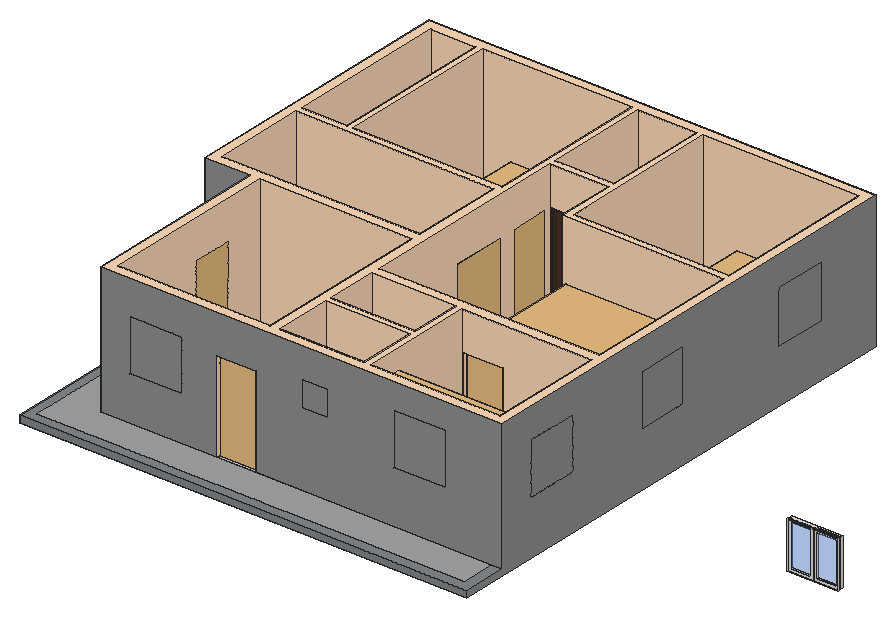
# SketchUp Ruby script. Lengths in inches.
U = 1.inch
M = Sketchup.active_model
def pt(a) = Geom::Point3d.new(a.map { |v| v * U })
def face(e, loops, mat)
  f = e.add_face(loops[0].map { |a| pt(a) })
  loops[1..].each { |l| e.add_face(l.map { |a| pt(a) }).erase! }
  f.material = f.back_material = mat if mat
  f
end
# faces: each face lists its corners as indices into pts; further lists are holes
def faces(e, pts, list, mat = nil) = list.each { |f| face(e, (f[0].is_a?(Array) ? f : [f]).map { |l| l.map { |i| pts[i] } }, mat) }
# xy, xz, yz: faces in a plane at the given z, y or x. An outline is a flat list of corners, or four numbers for a rectangle; further outlines are holes
def ring(l) = l.size == 4 ? [[l[0], l[1]], [l[2], l[1]], [l[2], l[3]], [l[0], l[3]]] : l.each_slice(2).to_a
def flat(e, list, mat, &to3) = list.each { |f| face(e, (f[0].is_a?(Array) ? f : [f]).map { |l| ring(l).map { |u, v| to3.(u, v) } }, mat) }
def xy(e, z, list, mat = nil) = flat(e, list, mat) { |x, y| [x, y, z] }
def xz(e, y, list, mat = nil) = flat(e, list, mat) { |x, z| [x, y, z] }
def yz(e, x, list, mat = nil) = flat(e, list, mat) { |y, z| [x, y, z] }
def lines(e, pts, list) = list.each { |a, b| e.add_line(pt(pts[a]), pt(pts[b])) }
# prism: a flat outline (further loops are holes) pulled along v
def prism(e, loops, v, mat = nil)
  f = face(e, loops, mat); d = Geom::Vector3d.new(v.map { |x| x * U })
  f.pushpull(f.normal.samedirection?(d) ? d.length : -d.length)
end
def box(e, o, s, mat = nil) = prism(e, [[o, [o[0] + s[0], o[1], o[2]], [o[0] + s[0], o[1] + s[1], o[2]], [o[0], o[1] + s[1], o[2]]]], [0, 0, s[2]], mat)
def at(x, y, z, deg = 0) = Geom::Transformation.translation(pt([x, y, z])) * Geom::Transformation.rotation(ORIGIN, Z_AXIS, deg.degrees)
def axes(o, x, y, z) = Geom::Transformation.new([*x, 0, *y, 0, *z, 0, *pt(o).to_a, 1])
def part(name) = M.definitions.add(name)
# library, detail: a bought-in or finely detailed component or shape, given as its bounding box
def library(name, o, s) = part(name).tap { |d| box(d.entities, o, s) }
def detail(e, o, s) = box(e.add_group.entities, o, s)
def put(e, d, t, mat = nil) = e.add_instance(d, t).tap { |i| i.material = mat if mat }
def group(e, t, mat = nil) = e.add_group.tap { |g| g.transformation = t; g.material = mat if mat }.entities
root = M.entities
M.materials.add("Polis06_194").color = [79, 50, 36]
M.materials.add("[0027_PeachPuff]").color = [255, 218, 185]
M.materials.add("[Blacktop Old 01]").color = [132, 136, 139]
M.materials.add("[Blacktop Old 02]").color = [143, 145, 145]
M.materials.add("[Marble Carrara Floor Tile]").color = [204, 208, 219]
M.materials.add("[Marble Carrara Floor Tile]1").color = [204, 208, 219]
M.materials.add("[Stone Vein Gray]").color = [166, 165, 165]
M.materials.add("[Translucent Glass Blue]").color = [100, 149, 237]
M.materials["[Translucent Glass Blue]"].alpha = 0.5
c1 = part("Flush door")
xy(c1.entities,0,[[0,0,4.72,1.18],[0,34.25,4.72,35.43]],"Polis06_194")
xy(c1.entities,85.26,[[0,1.18,4.72,34.25]],"Polis06_194")
xy(c1.entities,86.61,[[0,0,4.72,35.43]],"Polis06_194")
xz(c1.entities,0,[[0,0,4.72,86.61]],"Polis06_194")
xz(c1.entities,1.18,[[0,0,2.36,85.26],[2.36,0,4.72,85.26]],"Polis06_194")
xz(c1.entities,34.25,[[0,0,4.72,85.26]],"Polis06_194")
xz(c1.entities,35.43,[[0,0,4.72,86.61]],"Polis06_194")
yz(c1.entities,0,[[0,0,1.18,86.61],[34.25,0,35.43,86.61],[1.18,85.26,34.25,86.61]],"Polis06_194")
yz(c1.entities,2.36,[[1.18,0,34.25,0,34.25,85.21,1.18,85.26]],"Polis06_194")
yz(c1.entities,4.72,[[0,0,1.18,86.61],[34.25,0,35.43,86.61],[1.18,85.26,34.25,86.61]],"Polis06_194")
c2 = library("04+Sofa+y+Mesas (1)",[-94.93,-111.67,3.93],[153.81,110.61,64.28])
c3 = part("Janela aluminio")
xy(c3.entities,0,[[0,0,47.24,1.57],[23.62,1.57,47.24,2.76],[0,2.76,25.98,3.9375],[0,3.9375,47.24,5.91]])
xy(c3.entities,43.31,[[0,0,47.24,1.57],[23.62,1.57,47.24,2.76],[0,2.76,0,5.91,47.24,5.91,47.24,3.9375,25.98,3.9375,25.98,2.76],[25.98,2.76,47.24,3.9375]])
xz(c3.entities,1.57,[[0,0,23.62,0,23.62,41.34,21.26,41.34,21.26,1.97,1.97,1.97,1.97,41.34,23.62,41.34,23.62,43.31,0,43.31],[[23.62,0,47.24,43.31],[25.7,1.97,45.28,41.34]]])
xz(c3.entities,2.76,[[[0,0,23.62,43.31],[2.36,2.36,21.26,40.94]],[23.62,0,25.98,43.31]])
xz(c3.entities,2.76,[[2.36,2.36,21.26,40.94]],"[Translucent Glass Blue]")
xz(c3.entities,3.9375,[[25.98,0,25.98,2.36,44.88,2.36,44.88,40.94,25.98,40.94,25.98,43.31,47.24,43.31,47.24,0]])
xz(c3.entities,3.9375,[[25.98,2.36,44.88,40.94]],"[Translucent Glass Blue]")
yz(c3.entities,0,[[0,0,1.57,43.31],[2.76,0,5.91,43.31]])
yz(c3.entities,23.62,[[1.57,0,2.76,43.31]])
yz(c3.entities,25.98,[[2.76,0,3.9375,43.31]])
yz(c3.entities,47.24,[[0,0,1.57,43.31],[1.57,0,2.76,43.31],[3.9375,0,5.91,43.31]])
c4 = library("Interior door assembly",[0,0,0],[5.9375,43.31,84.65])
c5 = library("Double bed",[0,0,0],[83.59,95.6,35.43])
c6 = library("TS396-4",[-0.02,-3.5,-3.5],[8.95,7,28.74])
c7 = library("K-3457 - Kohler Devonshire(R) elongated toilet with left-han",[-8.99,-6.22,0],[17.99,30.87,31.5])
c8 = library("30\" Kohler Jacquard Vanity",[0,0,0],[30,21.875,40.63])
c9 = library("Group\#21",[0,-0.9375,0],[191.71,31.89,101.93])
xy(root,0,[[0,0,414,474]])
xy(root,6,[[0,0,414,0,414,41,405,41,405,9,9,9,9,214,0,214]],"[Blacktop Old 01]")
xy(root,6,[[150,41,186,41,186,50,192,50,192,52,201,52,201,50,279,50,279,103,201,103,201,82,192,82,192,109,279,109,279,156,201,156,201,139,192,139,192,214,190,214,190,223,154,223,154,214,51,214,51,176.66,42,176.66,42,140.66,51,140.66,51,50,150,50],[285,50,405,50,405,156,323,156,323,165,405,165,405,309,255,309,255,321,261,321,261,315,405,315,405,465,261,465,261,357,255,357,255,363,233,363,233,369,255,369,255,465,201,465,201,369,203,369,203,363,201,363,201,357,195,357,195,465,57,465,57,357,51,357,51,465,9,465,9,315,51,315,51,321,57,321,57,315,195,315,195,321,201,321,201,303,192,303,192,255,201,255,201,165,287,165,287,156,285,156]],"[Marble Carrara Floor Tile]")
xy(root,6,[[9,223,51,309],[51,223,151,309],[151,223,192,309]],"[Marble Carrara Floor Tile]1")
xy(root,6,[[9,9,405,9,405,41,42,41,42,214,9,214]],"[Stone Vein Gray]")
xy(root,90,[[150,41,186,50],[192,52,201,82],[192,109,201,139],[42,140.66,51,176.66],[287,156,323,165],
  [154,214,190,223],[192,255,201,303],[51,321,57,357],[195,321,201,357],[255,321,261,357],
  [203,363,233,369]])
xy(root,126,[[[42,41,414,41,414,474,0,474,0,214,42,214],[201,165,201,363,255,363,255,309,405,309,405,165],[51,50,192,214],[261,315,405,465],[57,315,195,465],[9,223,192,309],[285,50,405,156],[9,315,51,465],[201,369,255,465],[201,50,279,103],[201,109,279,156]]],"[0027_PeachPuff]")
xz(root,0,[[0,0,414,6]],"[Blacktop Old 01]")
xz(root,41,[[[42,6,150,6,150,90,186,90,186,6,414,6,414,126,42,126],[314.02,54.84,362.02,102.84],[69,46.6,117,94.6],[228.3,74.23,252.3,98.23]],[69,46.6,117,94.6],[314.02,54.84,362.02,102.84],[228.3,74.23,252.3,98.23]],"[Blacktop Old 02]")
xz(root,50,[[51,6,51,126,192,126,192,6,186,6,186,90,150,90,150,6],[201,6,279,126],[285,6,405,126]],"[0027_PeachPuff]")
xz(root,52,[[192,6,201,90]],"[0027_PeachPuff]")
xz(root,82,[[192,6,201,90]],"[0027_PeachPuff]")
xz(root,103,[[201,6,279,126]],"[0027_PeachPuff]")
xz(root,109,[[192,6,192,90,201,90,201,126,279,126,279,6]],"[0027_PeachPuff]")
xz(root,139,[[192,6,201,90]],"[0027_PeachPuff]")
xz(root,140.66,[[42,6,51,90]],"[0027_PeachPuff]")
xz(root,156,[[201,6,279,126],[285,6,287,6,287,90,323,90,323,6,405,6,405,126,285,126]],"[0027_PeachPuff]")
xz(root,165,[[201,6,201,126,405,126,405,6,323,6,323,90,287,90,287,6]],"[0027_PeachPuff]")
xz(root,176.66,[[42,6,51,90]],"[0027_PeachPuff]")
xz(root,214,[[51,6,154,6,154,90,190,90,190,6,192,6,192,126,51,126]],"[0027_PeachPuff]")
xz(root,214,[[0,6,42,126]],"[Blacktop Old 02]")
xz(root,223,[[9,6,9,126,192,126,192,6,190,6,190,90,154,90,154,6]],"[0027_PeachPuff]")
xz(root,255,[[192,6,201,90]],"[0027_PeachPuff]")
xz(root,303,[[192,6,201,90]],"[0027_PeachPuff]")
xz(root,309,[[9,6,192,126],[255,6,405,126]],"[0027_PeachPuff]")
xz(root,315,[[9,6,51,126],[57,6,195,126],[261,6,405,126]],"[0027_PeachPuff]")
xz(root,321,[[51,6,57,90],[195,6,201,90],[255,6,261,90]],"[0027_PeachPuff]")
xz(root,357,[[51,6,57,90],[195,6,201,90],[255,6,261,90]],"[0027_PeachPuff]")
xz(root,363,[[201,6,203,6,203,90,233,90,233,6,255,6,255,126,201,126]],"[0027_PeachPuff]")
xz(root,369,[[201,6,201,126,255,126,255,6,233,6,233,90,203,90,203,6]],"[0027_PeachPuff]")
xz(root,465,[[9,6,51,126],[57,6,195,126],[201,6,255,126],[261,6,405,126]],"[0027_PeachPuff]")
xz(root,474,[[[0,0,414,126],[104.07,47.27,152.07,95.27],[318.51,50.36,366.51,98.36],[217.61,68.5,241.61,92.5]],[104.07,47.27,152.07,95.27],[318.51,50.36,366.51,98.36],[217.61,68.5,241.61,92.5]],"[Blacktop Old 02]")
yz(root,0,[[[0,0,0,6,214,6,214,126,474,126,474,0],[241.85,47.3,289.85,95.3]],[241.85,47.3,289.85,95.3]],"[Blacktop Old 02]")
yz(root,9,[[223,6,309,126],[315,6,465,126]],"[0027_PeachPuff]")
yz(root,42,[[[41,6,41,126,214,126,214,6,176.66,6,176.66,90,140.66,90,140.66,6],[68.36,45.06,116.36,93.06]],[68.36,45.06,116.36,93.06]],"[Blacktop Old 02]")
yz(root,51,[[50,6,140.66,6,140.66,90,176.66,90,176.66,6,214,6,214,126,50,126],[[315,6,315,126,465,126,465,6,357,6,357,90,321,90,321,6],[386.66,46.95,434.66,94.95]],[386.66,46.95,434.66,94.95]],"[0027_PeachPuff]")
yz(root,57,[[315,6,321,6,321,90,357,90,357,6,465,6,465,126,315,126]],"[0027_PeachPuff]")
yz(root,150,[[41,6,50,90]],"[0027_PeachPuff]")
yz(root,154,[[214,6,223,90]],"[0027_PeachPuff]")
yz(root,186,[[41,6,50,90]],"[0027_PeachPuff]")
yz(root,190,[[214,6,223,90]],"[0027_PeachPuff]")
yz(root,192,[[50,6,50,126,214,126,214,6,139,6,139,90,109,90,109,6,82,6,82,90,52,90,52,6],[223,6,223,126,309,126,309,6,303,6,303,90,255,90,255,6]],"[0027_PeachPuff]")
yz(root,195,[[315,6,315,126,465,126,465,6,357,6,357,90,321,90,321,6]],"[0027_PeachPuff]")
yz(root,201,[[50,6,52,6,52,90,82,90,82,6,103,6,103,126,50,126],[139,6,156,6,156,126,109,126,109,90,139,90],[165,6,255,6,255,90,303,90,303,6,321,6,321,90,357,90,357,6,363,6,363,126,165,126],[369,6,465,126]],"[0027_PeachPuff]")
yz(root,203,[[363,6,369,90]],"[0027_PeachPuff]")
yz(root,233,[[363,6,369,90]],"[0027_PeachPuff]")
yz(root,255,[[309,6,309,126,363,126,363,6,357,6,357,90,321,90,321,6],[369,6,465,126]],"[0027_PeachPuff]")
yz(root,261,[[315,6,321,6,321,90,357,90,357,6,465,6,465,126,315,126]],"[0027_PeachPuff]")
yz(root,279,[[50,6,103,126],[109,6,156,126]],"[0027_PeachPuff]")
yz(root,285,[[50,6,156,126]],"[0027_PeachPuff]")
yz(root,287,[[156,6,165,90]],"[0027_PeachPuff]")
yz(root,323,[[156,6,165,90]],"[0027_PeachPuff]")
yz(root,405,[[50,6,156,126],[165,6,309,126],[315,6,465,126]],"[0027_PeachPuff]")
yz(root,414,[[[0,0,474,0,474,126,41,126,41,6,0,6],[361.74,50.31,409.74,98.31],[202.45,50.73,250.45,98.73],[74.57,50.35,122.57,98.35]],[361.74,50.31,409.74,98.31],[74.57,50.35,122.57,98.35],[202.45,50.73,250.45,98.73]],"[Blacktop Old 02]")
p = [[-53.125,398.49,-3.09],[-53.125,398.49,-0.9]]
lines(root,p,[[0,1]])
put(root,c1,axes([196.28,109,6],[1,0,0],[0,0.84667,0],[0,0,0.96982]))
put(root,c2,axes([349.0625,309.86,2.07],[0.95,0,0],[0,0.81,0],[0,0,1]))
put(root,c3,at(570.64,175.16,0))
put(root,c4,axes([45.0625,140.66,6],[1,0,0],[0,0.83127,0],[0,0,0.99237]))
put(root,c1,axes([196.28,52,6],[1,0,0],[0,0.84667,0],[0,0,0.96982]))
put(root,c1,axes([203,367.72,6],[0,-1,0],[0.84667,0,0],[0,0,0.96982]))
put(root,c4,axes([51.0625,321,6],[1,0,0],[0,0.83127,0],[0,0,0.99237]))
put(root,c4,axes([195.0625,321,6],[1,0,0],[0,0.83127,0],[0,0,0.99237]))
put(root,c4,axes([255.0625,321,6],[1,0,0],[0,0.83127,0],[0,0,0.99237]))
put(root,c4,axes([287,165,6],[0,-1,0],[0.83127,0,0],[0,0,0.99237]))
put(root,c4,axes([150,50,6],[0,-1,0],[0.83127,0,0],[0,0,0.99237]))
put(root,c4,axes([154,223,6],[0,-1,0],[0.83127,0,0],[0,0,0.99237]))
put(root,c4,axes([196.0625,255,6],[1,0,0],[0,1.10836,0],[0,0,0.99237]))
put(root,c5,at(178.34,381.41,6,90))
put(root,c5,at(388.16,381.41,6,90))
put(root,c5,at(52.06,133.59,6,-90))
put(root,c6,axes([254.99,446.64,41.49],[-1,0,0],[0,1.1793,0],[0,0,1.85]))
put(root,c7,axes([249.1,417.89,6],[0,0.89,0],[-0.89,0,0],[0,0,0.89]))
put(root,c8,axes([239.47,400.86,6],[0,-0.71,0],[0.71,0,0],[0,0,0.71]))
put(root,c6,axes([271.14,50.01,41.49],[0,1,0],[1.1793,0,0],[0,0,1.85]))
put(root,c7,axes([242.38,55.9,6],[0.89,0,0],[0,0.89,0],[0,0,0.89]))
put(root,c8,axes([225.35,65.53,6],[-0.71,0,0],[0,-0.71,0],[0,0,0.71]))
put(root,c9,axes([405,80.95,6],[-0.6264,0,0],[0,-1,0],[0,0,1]))
